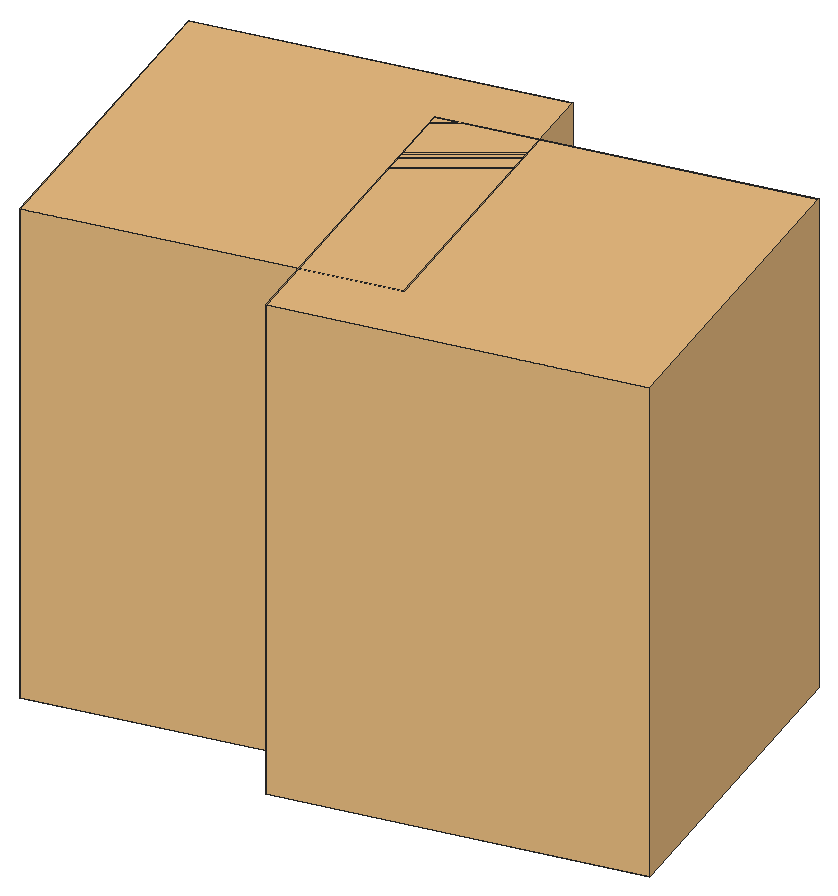
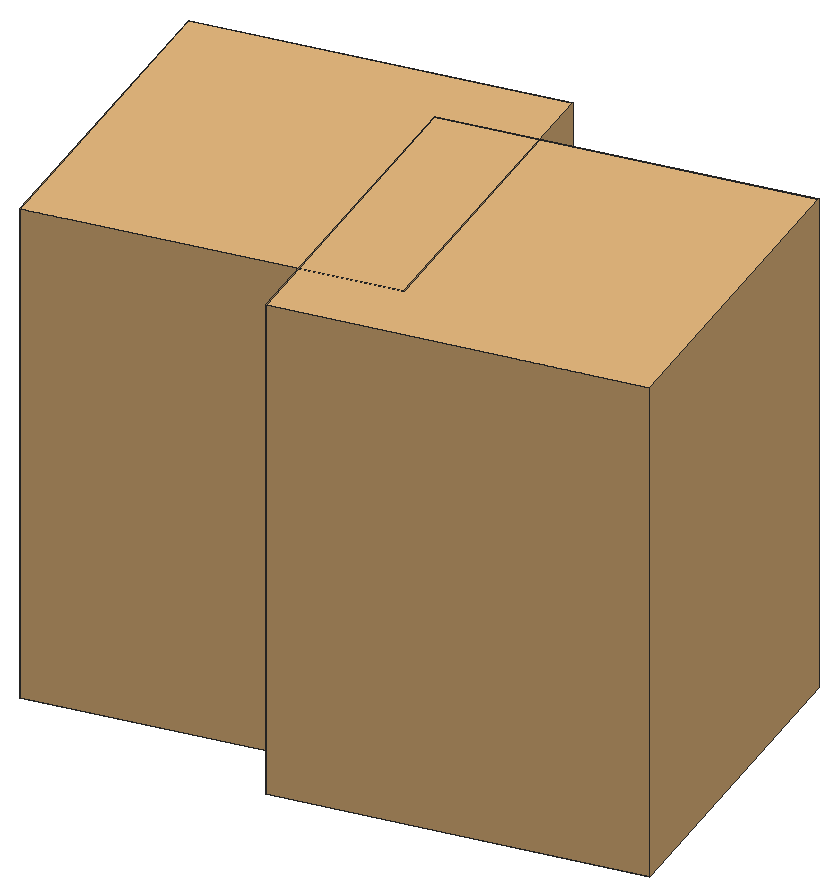
# SketchUp Ruby script. Lengths in inches.
U = 1.inch
M = Sketchup.active_model
def pt(a) = Geom::Point3d.new(a.map { |v| v * U })
def face(e, loops, mat)
  f = e.add_face(loops[0].map { |a| pt(a) })
  loops[1..].each { |l| e.add_face(l.map { |a| pt(a) }).erase! }
  f.material = f.back_material = mat if mat
  f
end
# faces: each face lists its corners as indices into pts; further lists are holes
def faces(e, pts, list, mat = nil) = list.each { |f| face(e, (f[0].is_a?(Array) ? f : [f]).map { |l| l.map { |i| pts[i] } }, mat) }
# xy, xz, yz: faces in a plane at the given z, y or x. An outline is a flat list of corners, or four numbers for a rectangle; further outlines are holes
def ring(l) = l.size == 4 ? [[l[0], l[1]], [l[2], l[1]], [l[2], l[3]], [l[0], l[3]]] : l.each_slice(2).to_a
def flat(e, list, mat, &to3) = list.each { |f| face(e, (f[0].is_a?(Array) ? f : [f]).map { |l| ring(l).map { |u, v| to3.(u, v) } }, mat) }
def xy(e, z, list, mat = nil) = flat(e, list, mat) { |x, y| [x, y, z] }
def xz(e, y, list, mat = nil) = flat(e, list, mat) { |x, z| [x, y, z] }
def yz(e, x, list, mat = nil) = flat(e, list, mat) { |y, z| [x, y, z] }
def lines(e, pts, list) = list.each { |a, b| e.add_line(pt(pts[a]), pt(pts[b])) }
# prism: a flat outline (further loops are holes) pulled along v
def prism(e, loops, v, mat = nil)
  f = face(e, loops, mat); d = Geom::Vector3d.new(v.map { |x| x * U })
  f.pushpull(f.normal.samedirection?(d) ? d.length : -d.length)
end
def box(e, o, s, mat = nil) = prism(e, [[o, [o[0] + s[0], o[1], o[2]], [o[0] + s[0], o[1] + s[1], o[2]], [o[0], o[1] + s[1], o[2]]]], [0, 0, s[2]], mat)
def at(x, y, z, deg = 0) = Geom::Transformation.translation(pt([x, y, z])) * Geom::Transformation.rotation(ORIGIN, Z_AXIS, deg.degrees)
def axes(o, x, y, z) = Geom::Transformation.new([*x, 0, *y, 0, *z, 0, *pt(o).to_a, 1])
def part(name) = M.definitions.add(name)
# library, detail: a bought-in or finely detailed component or shape, given as its bounding box
def library(name, o, s) = part(name).tap { |d| box(d.entities, o, s) }
def detail(e, o, s) = box(e.add_group.entities, o, s)
def put(e, d, t, mat = nil) = e.add_instance(d, t).tap { |i| i.material = mat if mat }
def group(e, t, mat = nil) = e.add_group.tap { |g| g.transformation = t; g.material = mat if mat }.entities
root = M.entities
M.materials.add("Material82").color = [68, 110, 58]
M.materials.add("Material83").color = [48, 90, 38]
M.materials.add("Material84").color = [68, 110, 48]
M.materials.add("Material85").color = [48, 90, 48]
M.materials.add("Material86").color = [58, 110, 58]
M.materials.add("Material87").color = [58, 90, 38]
M.materials.add("Material88").color = [68, 100, 58]
M.materials.add("Material89").color = [48, 100, 38]
c1 = part("grass00")
p = [[-0.6875,0.15,0],[-0.56,0.08,5.52],[-0.04,0.03,2.76],[0.48,-0.02,0],[0.35,-0.02,5.52],[-0.1,-0.14,5.52],
  [-0.12,0.65,8.37],[-0.42,0.65,8.37]]
faces(c1.entities,p,[[0,1,2,3],[3,2,4],[1,5,2],[5,4,2],[1,6,5],[4,5,6],[7,6,1]])
c2 = part("Group16\#1")
put(c2.entities,c1,axes([1.44,-0.61,-0.01],[0.05352,0.12609,0],[-0.10704,0.04543,0.07239],[0.06664,-0.02828,0.11628]),"Material85")
put(c2.entities,c1,axes([0.76,-0.15,-0.01],[0.04676,0.24062,0],[-0.23162,0.04501,0.06642],[0.0652,-0.01267,0.23595]),"Material82")
put(c2.entities,c1,axes([0.79,0.01,-0.01],[-0.00606,0.34651,0],[-0.34381,-0.00602,0.0432],[0.04319,0.00076,0.34386]))
put(c2.entities,c1,axes([1,0.23,-0.01],[-0.07192,0.31144,0],[-0.28722,-0.06632,0.1236],[0.12043,0.02781,0.29478]),"Material84")
put(c2.entities,c1,axes([1.66,0.77,-0.01],[-0.13828,0.29651,0],[-0.21551,-0.1005,0.22471],[0.20365,0.09498,0.23779]),"Material89")
put(c2.entities,c1,axes([0.6875,0.52,-0.01],[-0.18126,0.24051,0],[-0.22746,-0.17142,0.09788],[0.07817,0.05891,0.28481]),"Material84")
put(c2.entities,c1,axes([0.68,0.78,-0.01],[-0.215,0.18688,0],[-0.12385,-0.14248,0.21334],[0.13995,0.16101,0.18878]),"Material82")
put(c2.entities,c1,axes([0.56,1,-0.01],[-0.13756,0.07624,0],[-0.06159,-0.11112,0.0927],[0.04494,0.08108,0.12705]),"Material84")
put(c2.entities,c1,axes([0.2,0.64,-0.01],[-0.23729,0.07254,0],[-0.05711,-0.18681,0.153],[0.04473,0.14632,0.19535]),"Material89")
put(c2.entities,c1,axes([0.0625,0.72,-0.01],[-0.28874,0.02525,0],[-0.02179,-0.24916,0.14647],[0.01276,0.14591,0.25012]),"Material82")
put(c2.entities,c1,axes([-0.08,0.62,-0.01],[-0.34089,-0.04187,0],[0.03255,-0.26504,0.216],[-0.02633,0.21439,0.26703]),"Material89")
put(c2.entities,c1,axes([-0.34,0.98,-0.01],[-0.14314,-0.0493,0],[0.04397,-0.12769,0.06843],[-0.02228,0.0647,0.13505]),"Material89")
put(c2.entities,c1,axes([-0.87,1.45,-0.01],[-0.23488,-0.14114,0],[0.13761,-0.22901,0.06087],[-0.03135,0.05217,0.26717]))
put(c2.entities,c1,axes([-0.72,0.77,-0.01],[-0.14208,-0.13251,0],[0.07209,-0.0773,0.16301],[-0.11118,0.11922,0.1057]),"Material89")
put(c2.entities,c1,axes([-0.62,0.43,-0.01],[-0.14845,-0.21203,0],[0.18654,-0.13061,0.12304],[-0.10079,0.07057,0.22772]),"Material82")
put(c2.entities,c1,axes([-0.68,0.29,-0.01],[-0.13639,-0.32136,0],[0.31723,-0.13464,0.05579],[-0.05136,0.0218,0.34462]),"Material83")
put(c2.entities,c1,axes([-0.64,0.125,-0.01],[-0.0458,-0.23569,0],[0.22124,-0.043,0.08276],[-0.08124,0.01579,0.22538]),"Material86")
put(c2.entities,c1,axes([-1.6,-0.03,-0.01],[0.00576,-0.32897,0],[0.27526,0.00482,0.18018],[-0.18015,-0.00315,0.2753]),"Material84")
put(c2.entities,c1,axes([-1.36,-0.31,-0.01],[0.05718,-0.24765,0],[0.18172,0.04196,0.17267],[-0.16825,-0.03885,0.1865]),"Material89")
put(c2.entities,c1,axes([-1.54,-0.72,-0.01],[0.06537,-0.14017,0],[0.13555,0.06321,0.03939],[-0.0357,-0.01665,0.14956]))
put(c2.entities,c1,axes([-1.19,-0.9,-0.01],[0.09597,-0.12735,0],[0.11214,0.08451,0.07557],[-0.06035,-0.04548,0.14042]),"Material88")
put(c2.entities,c1,axes([-0.47,-0.54,-0.01],[0.11588,-0.10072,0],[0.0618,0.0711,0.12124],[-0.07953,-0.0915,0.0942]))
put(c2.entities,c1,axes([-0.47,-0.84,-0.01],[0.11927,-0.0661,0],[0.06603,0.11913,0.00646],[-0.00313,-0.00565,0.13621]),"Material84")
put(c2.entities,c1,axes([-0.38,-1.24,-0.01],[0.28037,-0.08571,0],[0.0618,0.20215,0.20315],[-0.05939,-0.19428,0.21139]),"Material88")
put(c2.entities,c1,axes([-0.06,-0.66,-0.01],[0.22719,-0.01987,0],[0.01247,0.14255,0.17758],[-0.01547,-0.17691,0.1431]),"Material87")
put(c2.entities,c1,axes([0.11,-0.89,-0.01],[0.14882,0.01828,0],[-0.01058,0.08611,0.12229],[0.01491,-0.12138,0.08676]),"Material85")
put(c2.entities,c1,axes([0.25,-0.72,-0.01],[0.20481,0.07053,0],[-0.06206,0.18022,0.10291],[0.03351,-0.0973,0.1906]),"Material85")
put(c2.entities,c1,axes([0.85,-1.42,-0.01],[0.16481,0.09904,0],[-0.09472,0.15762,0.05616],[0.02893,-0.04814,0.18389]),"Material84")
put(c2.entities,c1,axes([1.01,-1.09,-0.01],[0.21858,0.20385,0],[-0.17495,0.1876,0.15339],[0.10462,-0.11218,0.25652]),"Material89")
put(c2.entities,c1,axes([1.01,-0.71,-0.01],[0.08733,0.12473,0],[-0.06445,0.04512,0.13037],[0.1068,-0.07477,0.07867]),"Material85")
c3 = part("Group15\#1")
put(c3.entities,c2,at(0,0,0))
c4 = part("3darcstudiotree_grass00\#1")
put(c4.entities,c3,at(0,0,0))
c5 = library("Palm tree",[-4.09,-4.52,0],[193.52,193.51,258.93])
c6 = part("Palm+Tree")
put(c6.entities,c5,at(25.51,-21.81,0,15))
c7 = library("Group\#612",[0,0,0],[32.91,53.52,103.45])
put(root,c4,axes([808,966.58,-29.74],[3.38368,1.04745,0],[-2.27938,1.14521,-0.02005],[-0.08327,0.04184,1.86077]))
put(root,c4,axes([810.05,994.28,-29.74],[0.01113,-1.45353,0],[4.54919,0.00542,-0.03692],[0.17089,0.0002,1.57831]))
put(root,c4,axes([810.38,972.38,-29.74],[-1.2969,-1.20265,0],[3.80092,-0.63749,-0.01791],[0.10113,-0.01696,1.89984]))
put(root,c4,axes([810.49,950.74,-29.74],[0.25593,-1.38573,0],[3.33259,0.09573,-0.00937],[0.07232,0.00208,1.93766]))
put(root,c4,axes([810.38,946.16,-29.74],[-3.13946,0.49629,0],[-1.50487,-1.48058,-0.04281],[-0.09532,-0.09378,1.81418]))
put(root,c4,axes([810.27,988.9,-29.74],[3.11316,-1.08854,0],[2.76667,1.23063,-0.03392],[0.0954,0.04244,1.32537]))
put(root,c4,axes([811.375,957.3,-29.74],[-3.90762,0.14516,0],[-0.37668,-1.57704,-0.0202],[-0.01231,-0.05153,1.95637]))
put(root,c4,axes([810.23,941.52,-29.74],[3.63772,-0.04618,0],[0.1059,1.29755,-0.04101],[0.00733,0.08987,1.37186]))
put(root,c4,axes([810.3,996.94,-29.74],[0.13497,1.53866,0],[-3.75353,0.05121,-0.02489],[-0.17047,0.00233,1.9295]))
put(root,c4,axes([810.86,992.46,-29.74],[-2.50392,0.92561,0],[-3.00944,-1.26617,-0.02311],[-0.06646,-0.02796,1.38694]))
put(root,c4,axes([812.01,985.73,-29.74],[-4.13167,0.24366,0],[-0.69238,-1.82599,-0.06496],[-0.05165,-0.1362,1.88637]))
put(root,c4,axes([811.21,968.625,-29.74],[-1.70819,1.11812,0],[-3.96876,-0.943,-0.04504],[-0.21667,-0.05148,1.9506]))
put(root,c4,axes([811.39,977.74,-29.74],[3.79912,-1.05543,0],[2.19489,1.22878,-0.03692],[0.13668,0.07652,1.83631]))
put(root,c4,axes([811.27,943.99,-29.74],[3.28657,0.21022,0],[-0.53923,1.31117,-0.01255],[-0.01302,0.03166,1.63564]))
put(root,c4,axes([811.87,983.93,-29.74],[-2.37455,1.29783,0],[-2.73236,-0.77752,-0.00844],[-0.03827,-0.01089,1.41311]))
put(root,c4,axes([811.19,974.99,-29.74],[2.3712,1.21069,0],[-3.58151,1.09097,-0.04605],[-0.15475,0.04714,1.44046]))
put(root,c4,axes([812.42,960.11,-29.74],[1.66455,-1.14728,0],[3.31311,0.74761,-0.04415],[0.26641,0.06012,1.98924]))
put(root,c4,axes([813.52,990.33,-29.74],[-0.63027,-1.58552,0],[4.65732,-0.28794,-0.06318],[0.24644,-0.01524,1.39517]))
put(root,c4,axes([811.98,961.55,-29.74],[2.52471,1.58546,0],[-3.52346,0.87265,-0.052],[-0.25077,0.06211,1.7759]))
put(root,c4,axes([812.76,982.34,-29.74],[3.33412,-1.28398,0],[2.96352,1.19685,-0.04175],[0.14903,0.06019,1.62422]))
put(root,c4,axes([812.16,978.86,-29.74],[3.98735,0.11869,0],[-0.3473,1.81468,-0.00004],[-0.00002,0.00009,1.93334]))
put(root,c4,axes([813.8,953.3125,-29.74],[-2.08457,-1.53905,0],[3.84719,-0.81044,-0.05822],[0.30315,-0.06386,1.92982]))
put(root,c4,axes([812.93,970.21,-29.74],[0.24653,1.78059,0],[-4.18646,0.09015,-0.05861],[-0.36644,0.00789,1.96776]))
put(root,c4,axes([812.44,964.86,-29.74],[4.09909,0.70116,0],[-1.55013,1.40946,-0.01845],[-0.03388,0.03081,1.34771]))
put(root,c4,axes([812.47,940.48,-29.74],[1.95248,1.61036,0],[-3.842,0.72449,-0.01048],[-0.04175,0.00787,1.40926]))
put(root,c4,axes([812.8,955.24,-29.74],[3.93599,0.37319,0],[-1.10472,1.81211,-0.03506],[-0.03066,0.05029,1.32515]))
put(root,c4,axes([813.45,948.9,-29.74],[3.76504,-0.34797,0],[1.07827,1.81452,-0.02268],[0.0226,0.03802,1.5468]))
put(root,c4,axes([813.44,965.91,-29.74],[-0.03028,1.81071,0],[-4.52004,-0.01176,-0.01347],[-0.05788,-0.00015,1.45625]))
put(root,c4,axes([815.66,947.37,-29.74],[2.88127,-0.83898,0],[2.47269,1.32072,-0.02283],[0.06307,0.03369,1.4512]))
put(root,c4,axes([816.57,952.36,-29.74],[-1.69688,-1.72936,0],[4.23511,-0.64631,-0.05475],[0.2829,-0.04317,1.88574]))
put(root,c4,axes([815.66,944.48,-29.74],[3.22121,-0.88629,0],[2.07064,1.17047,-0.00731],[0.02777,0.0157,1.80073]))
put(root,c4,axes([816.79,994.51,-29.74],[-1.90792,-1.42621,0],[3.47826,-0.72369,-0.03938],[0.16408,-0.03414,1.38871]))
put(root,c4,axes([815.85,981.1,-29.74],[3.56261,-0.94567,0],[1.87037,1.0959,-0.0013],[0.00431,0.00253,1.49257]))
put(root,c4,axes([815.75,955.86,-29.74],[-1.05565,1.36177,0],[-3.91341,-0.47183,-0.0271],[-0.14616,-0.01762,1.72974]))
put(root,c4,axes([817.04,948.53,-29.74],[-4.0685,0.50795,0],[-1.17773,-1.46714,-0.03323],[-0.06082,-0.07576,1.77353]))
put(root,c4,axes([816.11,941.89,-29.74],[4.25936,0.17724,0],[-0.36955,1.38123,-0.03171],[-0.02162,0.08082,1.71518]))
put(root,c4,axes([817.72,958.15,-29.74],[0.20903,-1.7077,0],[3.89534,0.07416,-0.00402],[0.01821,0.00035,1.3243]))
put(root,c4,axes([817.82,964.27,-29.74],[-3.49989,-0.62042,0],[1.34924,-1.18377,-0.02079],[0.0557,-0.04887,1.61237]))
put(root,c4,axes([817.08,966.43,-29.74],[-2.24971,1.27376,0],[-2.901,-0.79689,-0.01437],[-0.08541,-0.02346,1.91898]))
put(root,c4,axes([817.98,988.83,-29.74],[-2.13915,-1.27276,0],[3.26215,-0.85272,-0.05028],[0.27845,-0.07279,1.94898]))
put(root,c4,axes([816.85,992.79,-29.74],[4.02195,-0.32221,0],[0.68718,1.33408,-0.00331],[0.00405,0.00786,1.58887]))
put(root,c4,axes([816.34,979.09,-29.74],[4.32701,0.55712,0],[-1.36775,1.65217,-0.00124],[-0.00192,0.00232,1.65228]))
put(root,c4,axes([817.54,986.48,-29.74],[-1.63539,1.16071,0],[-3.40916,-0.74706,-0.05151],[-0.29339,-0.06429,1.90487]))
put(root,c4,axes([816.75,983.57,-29.74],[1.01762,1.37596,0],[-4.26505,0.49058,-0.00405],[-0.01582,0.00182,1.35389]))
put(root,c4,axes([819.04,975.45,-29.74],[-3.3697,-1.02042,0],[2.44227,-1.25434,-0.00705],[0.02625,-0.01348,1.8369]))
put(root,c4,axes([818.17,977.03,-29.74],[2.02024,-1.18426,0],[3.76291,0.99837,-0.06298],[0.20491,0.05437,1.33293]))
put(root,c4,axes([817.39,940.4,-29.74],[4.3094,-0.16311,0],[0.42718,1.75528,-0.01064],[0.00539,0.02213,1.77558]))
put(root,c4,axes([819.16,990.66,-29.74],[-2.95002,-1.42448,0],[3.56758,-1.14909,-0.03335],[0.13906,-0.04479,1.85855]))
put(root,c4,axes([818.58,971.42,-29.74],[0.35372,-1.85816,0],[4.64402,0.13749,-0.06273],[0.35272,0.01044,1.9684]))
put(root,c4,axes([818.17,950.38,-29.74],[-1.74852,1.13217,0],[-3.21789,-0.77293,-0.03041],[-0.12145,-0.02917,1.3205]))
put(root,c4,axes([819.5,969.18,-29.74],[-1.80602,-1.23313,0],[3.1704,-0.72217,-0.00817],[0.04009,-0.00913,1.55447]))
put(root,c4,axes([818.74,972.1,-29.74],[3.72507,-0.62439,0],[1.73357,1.60854,-0.00549],[0.00931,0.00864,1.44062]))
put(root,c4,axes([818.74,960.3,-29.74],[3.99736,-0.43263,0],[1.22188,1.75587,-0.05143],[0.05673,0.08152,1.44218]))
put(root,c4,axes([818.7,962.125,-29.74],[-0.70731,1.48216,0],[-4.42453,-0.32839,-0.01956],[-0.1033,-0.00767,1.8138]))
put(root,c4,axes([821.18,958,-29.74],[-4.33089,0.41445,0],[-1.11243,-1.80796,-0.06662],[-0.06204,-0.10083,1.39642]))
put(root,c4,axes([822.0625,948.14,-29.74],[-3.26976,-0.5137,0],[1.67175,-1.65498,-0.00121],[0.00254,-0.00252,1.92636]))
put(root,c4,axes([821.3,992.46,-29.74],[1.4091,-1.17417,0],[3.00858,0.56155,-0.04441],[0.31581,0.05895,1.96303]))
put(root,c4,axes([822.04,988.18,-29.74],[-0.33318,-1.39627,0],[3.47077,-0.12881,-0.04952],[0.2452,-0.0091,1.29958]))
put(root,c4,axes([822.15,983.83,-29.74],[-3.53744,1.16554,0],[-2.5606,-1.20869,-0.03098],[-0.10582,-0.04995,1.59479]))
put(root,c4,axes([822.76,996.27,-29.74],[-3.84526,-0.22431,0],[0.50015,-1.33348,-0.00812],[0.00644,-0.01718,1.3892]))
put(root,c4,axes([822.28,978.95,-29.74],[-3.00421,0.76942,0],[-2.15411,-1.30812,-0.04277],[-0.14646,-0.08894,1.86401]))
put(root,c4,axes([821.75,950.6,-29.74],[-0.58592,1.57945,0],[-3.44253,-0.19862,-0.02144],[-0.15876,-0.00916,1.9513]))
put(root,c4,axes([822.26,971.43,-29.74],[-3.04736,0.88871,0],[-2.40783,-1.28411,-0.01371],[-0.03527,-0.01881,1.31321]))
put(root,c4,axes([821.75,990.875,-29.74],[3.34176,-0.01383,0],[0.04057,1.52455,-0.01029],[0.00052,0.01945,1.389]))
put(root,c4,axes([822.875,955.2,-29.74],[1.49416,-1.17809,0],[3.55261,0.70077,-0.01805],[0.08589,0.01694,1.58457]))
put(root,c4,axes([822,977.41,-29.74],[3.91979,-0.74164,0],[1.60866,1.32236,-0.04597],[0.11253,0.0925,1.57738]))
put(root,c4,axes([822.18,974.67,-29.74],[-2.1963,1.32957,0],[-3.96988,-1.01993,-0.00953],[-0.0332,-0.00853,1.47621]))
put(root,c4,axes([823.43,994.88,-29.74],[0.96851,-1.36822,0],[3.89034,0.4283,-0.00232],[0.01298,0.00143,1.76107]))
put(root,c4,axes([822.43,981.86,-29.74],[3.27047,-0.2692,0],[0.72961,1.37861,-0.04941],[0.05481,0.10356,1.4533]))
put(root,c4,axes([823.65,964.88,-29.74],[2.10515,-1.21949,0],[3.30844,0.88826,-0.01892],[0.09087,0.0244,1.74337]))
put(root,c4,axes([823.54,943.72,-29.74],[-2.16702,1.28274,0],[-3.03597,-0.79769,-0.03773],[-0.16249,-0.04269,1.41517]))
put(root,c4,axes([822.77,985.74,-29.74],[4.03817,0.43694,0],[-1.08149,1.5545,-0.02738],[-0.04454,0.06402,1.88342]))
put(root,c4,axes([823.32,972.08,-29.74],[4.33985,-0.71517,0],[1.81915,1.7169,-0.05614],[0.0962,0.09079,1.57175]))
put(root,c4,axes([824.33,960.42,-29.74],[1.94166,-1.68054,0],[3.68889,0.66287,-0.02827],[0.1643,0.02952,1.94019]))
put(root,c4,axes([823.64,966.31,-29.74],[0.75441,1.71197,0],[-3.26624,0.22386,-0.03272],[-0.2394,0.01641,1.8454]))
put(root,c4,axes([823.375,968.55,-29.74],[2.94946,0.97112,0],[-2.79078,1.31828,-0.05497],[-0.191,0.09022,1.76958]))
put(root,c4,axes([823.35,961.14,-29.74],[2.19107,1.06462,0],[-2.74426,0.87841,-0.00448],[-0.02021,0.00647,1.5389]))
put(root,c4,axes([824.5,953.46,-29.74],[2.33071,-1.20912,0],[3.74929,1.12403,-0.05929],[0.20074,0.06018,1.50135]))
put(root,c4,axes([824.25,942.1875,-29.74],[-0.50717,1.45325,0],[-4.1597,-0.22578,-0.0385],[-0.18859,-0.01024,1.55608]))
put(root,c4,axes([824.64,946.87,-29.74],[4.27397,-0.60338,0],[1.4489,1.5962,-0.05713],[0.08848,0.09748,1.48067]))
put(root,c4,axes([826.68,985.39,-29.74],[-2.9256,-1.47399,0],[3.63184,-1.12114,-0.01534],[0.06015,-0.01857,1.72134]))
put(root,c4,axes([826.47,970.86,-29.74],[-4.1987,0.12334,0],[-0.25997,-1.37638,-0.0204],[-0.0079,-0.04182,1.3669]))
put(root,c4,axes([826.84,990.07,-29.74],[-4.00085,-0.57986,0],[1.27846,-1.37193,-0.00277],[0.00474,-0.00509,1.38049]))
put(root,c4,axes([827.36,973.33,-29.74],[-3.39001,-0.81782,0],[2.4179,-1.55881,-0.03935],[0.08518,-0.05492,1.44076]))
put(root,c4,axes([826.68,946.19,-29.74],[3.84648,-0.75898,0],[1.52103,1.1989,-0.01525],[0.0428,0.03373,1.59832]))
put(root,c4,axes([827.3125,979.42,-29.74],[2.20697,-0.9726,0],[2.75858,0.97355,-0.01984],[0.09708,0.03426,1.82222]))
put(root,c4,axes([827.13,974.45,-29.74],[0.68368,1.71904,0],[-3.38759,0.20954,-0.03929],[-0.29518,0.01826,1.95437]))
put(root,c4,axes([828.6,981.53,-29.74],[-2.04632,-1.05436,0],[3.10393,-0.93693,-0.02737],[0.09658,-0.02915,1.30175]))
put(root,c4,axes([827.53,968.07,-29.74],[-0.28903,1.73584,0],[-3.34699,-0.08668,-0.03425],[-0.21957,-0.00569,1.61497]))
put(root,c4,axes([828.37,988.55,-29.74],[1.71259,-1.30416,0],[3.53393,0.72176,-0.01075],[0.04765,0.00973,1.48923]))
put(root,c4,axes([828.64,954.71,-29.74],[-3.772,0.03773,0],[-0.10384,-1.61464,-0.00196],[-0.00024,-0.00377,1.49745]))
put(root,c4,axes([827.98,949.1,-29.74],[-2.36342,1.1502,0],[-3.36153,-1.07427,-0.04128],[-0.15124,-0.04833,1.52936]))
put(root,c4,axes([827.56,953.5,-29.74],[4.05183,0.05747,0],[-0.14664,1.60785,-0.02702],[-0.00634,0.06949,1.99535]))
put(root,c4,axes([828.46,997.43,-29.74],[2.29885,-0.96399,0],[2.83055,1.04983,-0.02136],[0.08662,0.03213,1.62144]))
put(root,c4,axes([829.1875,951.28,-29.74],[-4.17405,-0.19289,0],[0.40333,-1.35747,-0.00847],[0.00693,-0.02334,1.82708]))
put(root,c4,axes([828.14,977.7,-29.74],[1.65421,1.20964,0],[-3.07102,0.65317,-0.03445],[-0.21317,0.04534,1.83855]))
put(root,c4,axes([829.84,945.24,-29.74],[-2.90823,-0.76432,0],[2.41266,-1.42777,-0.04785],[0.14851,-0.08788,1.82518]))
put(root,c4,axes([828.87,964.84,-29.74],[-1.04428,1.44728,0],[-3.25699,-0.36551,-0.00052],[-0.00331,-0.00037,1.67384]))
put(root,c4,axes([829,965.93,-29.74],[3.83018,0.17914,0],[-0.49889,1.65896,-0.05841],[-0.02825,0.09394,1.30397]))
put(root,c4,axes([830.52,959.08,-29.74],[-3.60335,-0.2844,0],[0.69529,-1.3701,-0.00178],[0.00231,-0.00455,1.75352]))
put(root,c4,axes([829.97,983.46,-29.74],[-2.93874,0.89671,0],[-2.33959,-1.1925,-0.04163],[-0.12402,-0.06321,1.39503]))
put(root,c4,axes([829.1,992.11,-29.74],[2.61631,0.861,0],[-2.17217,1.02658,-0.00812],[-0.03307,0.01563,1.6158]))
put(root,c4,axes([829.07,957.84,-29.74],[2.19518,1.25426,0],[-3.21279,0.87453,-0.02215],[-0.10628,0.02893,1.70619]))
put(root,c4,axes([829.74,941.48,-29.74],[0.43339,1.54675,0],[-3.36238,0.14653,-0.03685],[-0.25104,0.01094,1.73767]))
put(root,c4,axes([829.37,993.9375,-29.74],[3.82301,1.06562,0],[-2.5922,1.44638,-0.0169],[-0.04207,0.02347,1.45184]))
put(root,c4,axes([830.3125,961.87,-29.74],[3.73956,-0.25134,0],[0.58802,1.36068,-0.03176],[0.03776,0.08738,1.85682]))
put(root,c4,axes([832.18,954.85,-29.74],[-2.3605,-1.50274,0],[2.8114,-0.68684,-0.00146],[0.00663,-0.00162,1.32424]))
put(root,c4,axes([832.14,949.35,-29.74],[3.76532,-0.82989,0],[2.11238,1.49062,-0.04605],[0.09606,0.06778,1.38783]))
put(root,c4,axes([833.41,946.32,-29.74],[-2.75712,-0.97177,0],[2.36987,-1.04575,-0.04195],[0.16334,-0.07208,1.55746]))
put(root,c4,axes([831.98,992.35,-29.74],[1.13904,1.65719,0],[-4.07352,0.43546,-0.03421],[-0.20227,0.02162,1.93796]))
put(root,c4,axes([833.98,962.58,-29.74],[-1.0442,-1.68413,0],[4.42012,-0.42624,-0.03172],[0.12352,-0.01191,1.36741]))
put(root,c4,axes([834.13,942.29,-29.74],[-2.93582,-0.70247,0],[2.08855,-1.35755,-0.00574],[0.01328,-0.00863,1.3472]))
put(root,c4,axes([834.15,971.36,-29.74],[-2.87675,-1.09055,0],[2.6601,-1.09136,-0.02949],[0.13969,-0.05731,1.96656]))
put(root,c4,axes([834.3,976.82,-29.74],[-2.96111,-1.38906,0],[2.74036,-0.90856,-0.02964],[0.13819,-0.04582,1.63454]))
put(root,c4,axes([832.7,960.22,-29.74],[2.75422,1.28702,0],[-2.68657,0.89417,-0.05003],[-0.26479,0.08813,1.82479]))
put(root,c4,axes([832.87,966.43,-29.74],[2.36808,1.36159,0],[-2.95794,0.80011,-0.03781],[-0.20263,0.05481,1.74723]))
put(root,c4,axes([832.93,994.65,-29.74],[4.47082,0.11069,0],[-0.26321,1.65346,-0.04601],[-0.01202,0.07548,1.31249]))
put(root,c4,axes([833.57,975.17,-29.74],[-2.49032,1.32428,0],[-3.19574,-0.93467,-0.0152],[-0.05407,-0.01581,1.3203]))
put(root,c4,axes([833.02,967.68,-29.74],[1.04539,1.48143,0],[-4.29845,0.47176,-0.02844],[-0.1492,0.01637,1.82107]))
put(root,c4,axes([833.79,988.1875,-29.74],[-2.32252,1.56487,0],[-3.68383,-0.85034,-0.03733],[-0.14959,-0.03453,1.48568]))
put(root,c4,axes([833.18,983.05,-29.74],[2.07418,1.09295,0],[-3.13936,0.92662,-0.0157],[-0.06877,0.0203,1.60759]))
put(root,c4,axes([833.88,963.48,-29.74],[3.63146,-0.94763,0],[2.16895,1.29272,-0.03005],[0.10609,0.06323,1.88475]))
put(root,c4,axes([833.47,973.6,-29.74],[0.90968,1.754,0],[-3.81846,0.30801,-0.01369],[-0.06439,0.00519,1.40267]))
put(root,c4,axes([834.07,944.52,-29.74],[0.278,1.64734,0],[-3.85699,0.10123,-0.01024],[-0.06423,0.00169,1.82096]))
put(root,c4,axes([834.57,980.76,-29.74],[-1.2304,1.69187,0],[-3.83777,-0.43408,-0.02925],[-0.12783,-0.01446,1.36051]))
put(root,c4,axes([834.23,986.38,-29.74],[2.50159,1.07866,0],[-2.96417,1.06917,-0.03451],[-0.16033,0.05783,1.89576]))
put(root,c4,axes([834.38,990.76,-29.74],[3.85299,0.72056,0],[-1.4234,1.18377,-0.0026],[-0.00811,0.00675,1.81639]))
put(root,c4,axes([835.9375,953.26,-29.74],[-3.94572,0.20967,0],[-0.54102,-1.58348,-0.01091],[-0.00895,-0.02619,1.8656]))
put(root,c4,axes([834.58,950.24,-29.74],[4.67805,0.10708,0],[-0.2535,1.72242,-0.0212],[-0.00736,0.05004,1.96575]))
put(root,c4,axes([834.87,979,-29.74],[3.89819,0.51903,0],[-1.48599,1.73579,-0.0473],[-0.0826,0.09649,1.90097]))
put(root,c4,axes([834.93,997.3,-29.74],[3.72345,0.43237,0],[-1.05501,1.41306,-0.01058],[-0.0164,0.02196,1.53588]))
put(root,c4,axes([835.1,957.49,-29.74],[3.62609,0.38691,0],[-0.94095,1.37154,-0.04799],[-0.07441,0.10847,1.60328]))
put(root,c4,axes([838.19,946.9,-29.74],[-2.74827,-0.90606,0],[2.5057,-1.18207,-0.04185],[0.15974,-0.07536,1.7425]))
put(root,c4,axes([838.47,978.92,-29.74],[-2.21298,-1.13198,0],[3.27865,-0.99688,-0.03514],[0.15829,-0.04813,1.76492]))
put(root,c4,axes([838.41,990.26,-29.74],[1.56077,-1.21628,0],[3.51485,0.70149,-0.00728],[0.02929,0.00585,1.33141]))
put(root,c4,axes([837.89,992.375,-29.74],[-1.38329,1.54062,0],[-3.20389,-0.44741,-0.04758],[-0.27737,-0.03873,1.57537]))
put(root,c4,axes([838.94,951.05,-29.74],[-4.11808,-0.53305,0],[1.24091,-1.491,-0.0393],[0.07027,-0.08443,1.71017]))
put(root,c4,axes([838.51,982.05,-29.74],[-3.99092,0.85507,0],[-1.6879,-1.22527,-0.00649],[-0.01661,-0.01206,1.42064]))
put(root,c4,axes([837.86,994.9,-29.74],[-0.13254,1.67215,0],[-3.60359,-0.04442,-0.04056],[-0.20717,-0.00255,1.38085]))
put(root,c4,axes([838.72,961.12,-29.74],[-1.8566,1.22673,0],[-3.23788,-0.76215,-0.0186],[-0.08298,-0.01953,1.46845]))
put(root,c4,axes([838.89,972.03,-29.74],[3.63516,-0.37062,0],[1.04175,1.58916,-0.04398],[0.06662,0.10163,1.88821]))
put(root,c4,axes([838.84,942.59,-29.74],[4.38242,0.53414,0],[-1.34963,1.72221,-0.04987],[-0.06942,0.08859,1.61513]))
put(root,c6,at(783.23,891.52,-29.74))
put(root,c7,axes([950.92,894.49,-29.74],[1.13014,0.75656,0],[-0.75656,1.13014,0],[0,0,1.36]))
put(root,c6,at(928.6,891.52,-29.74))
